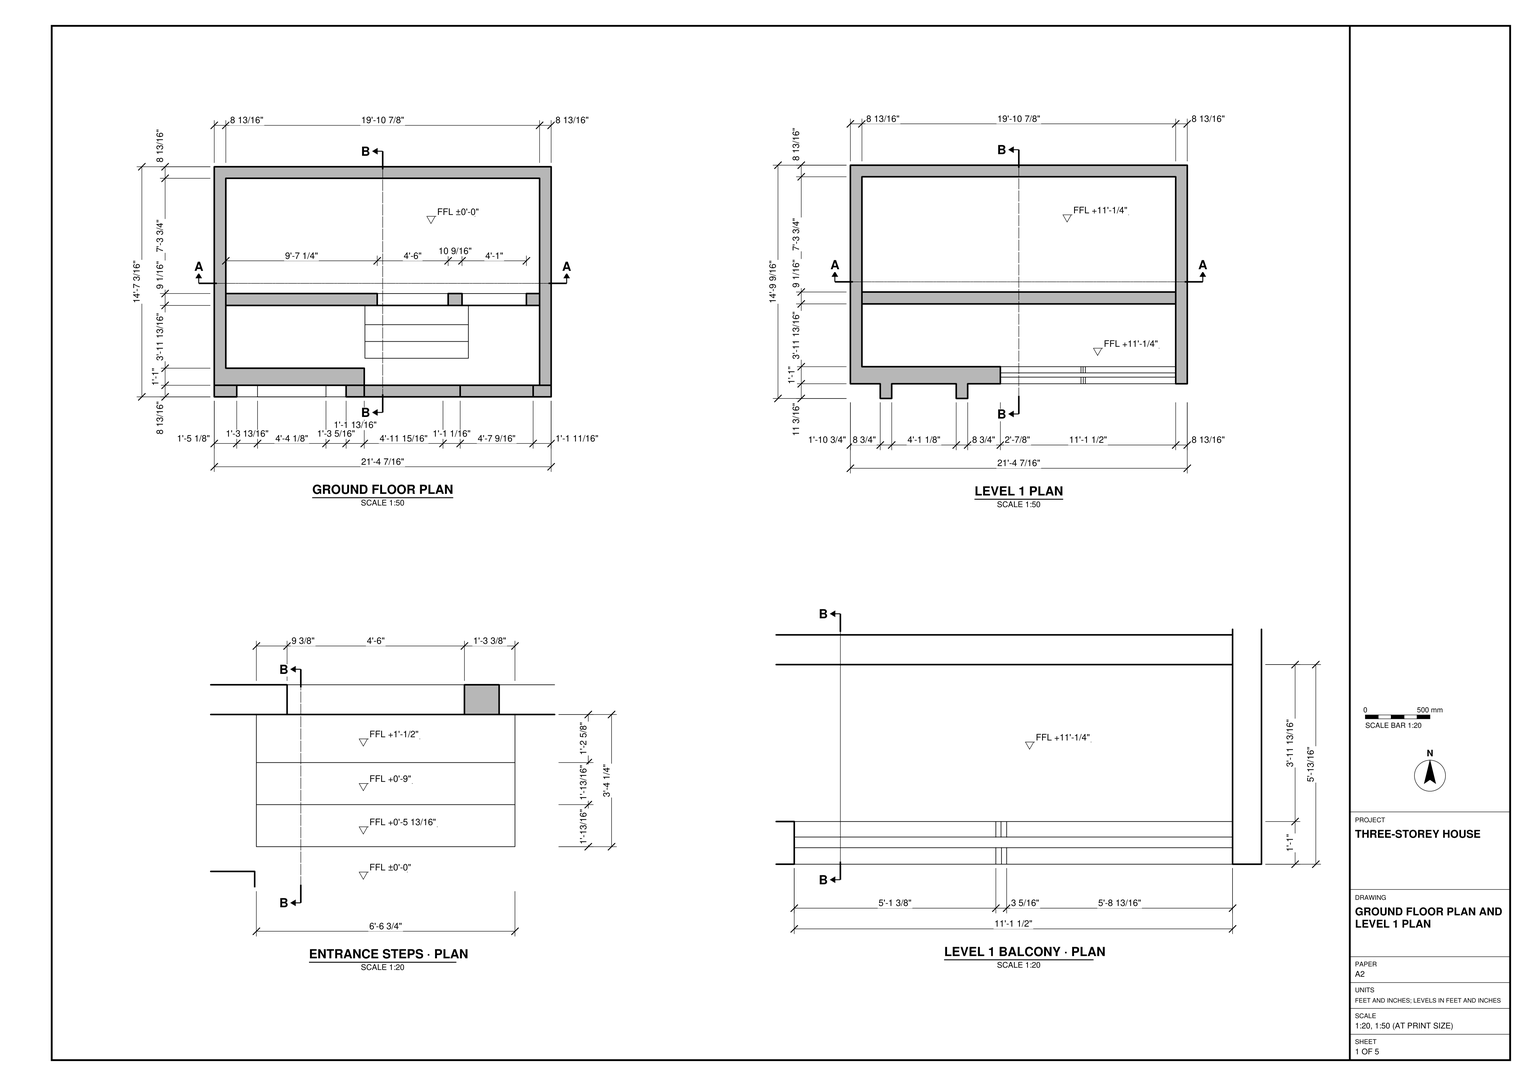
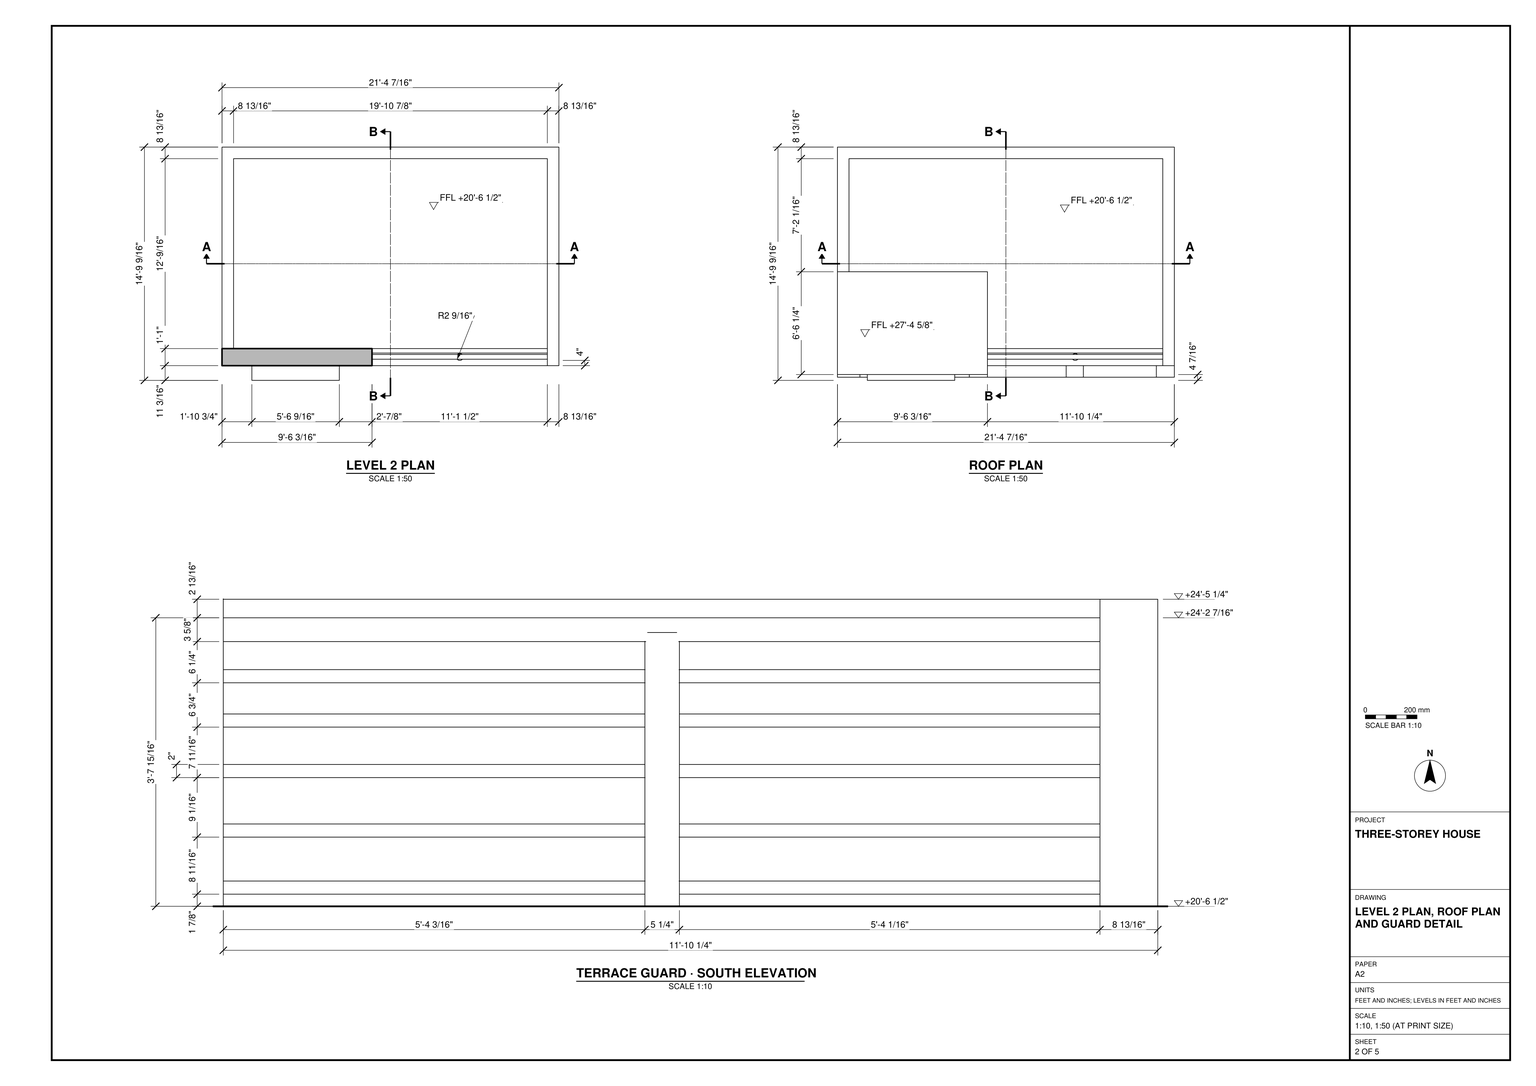
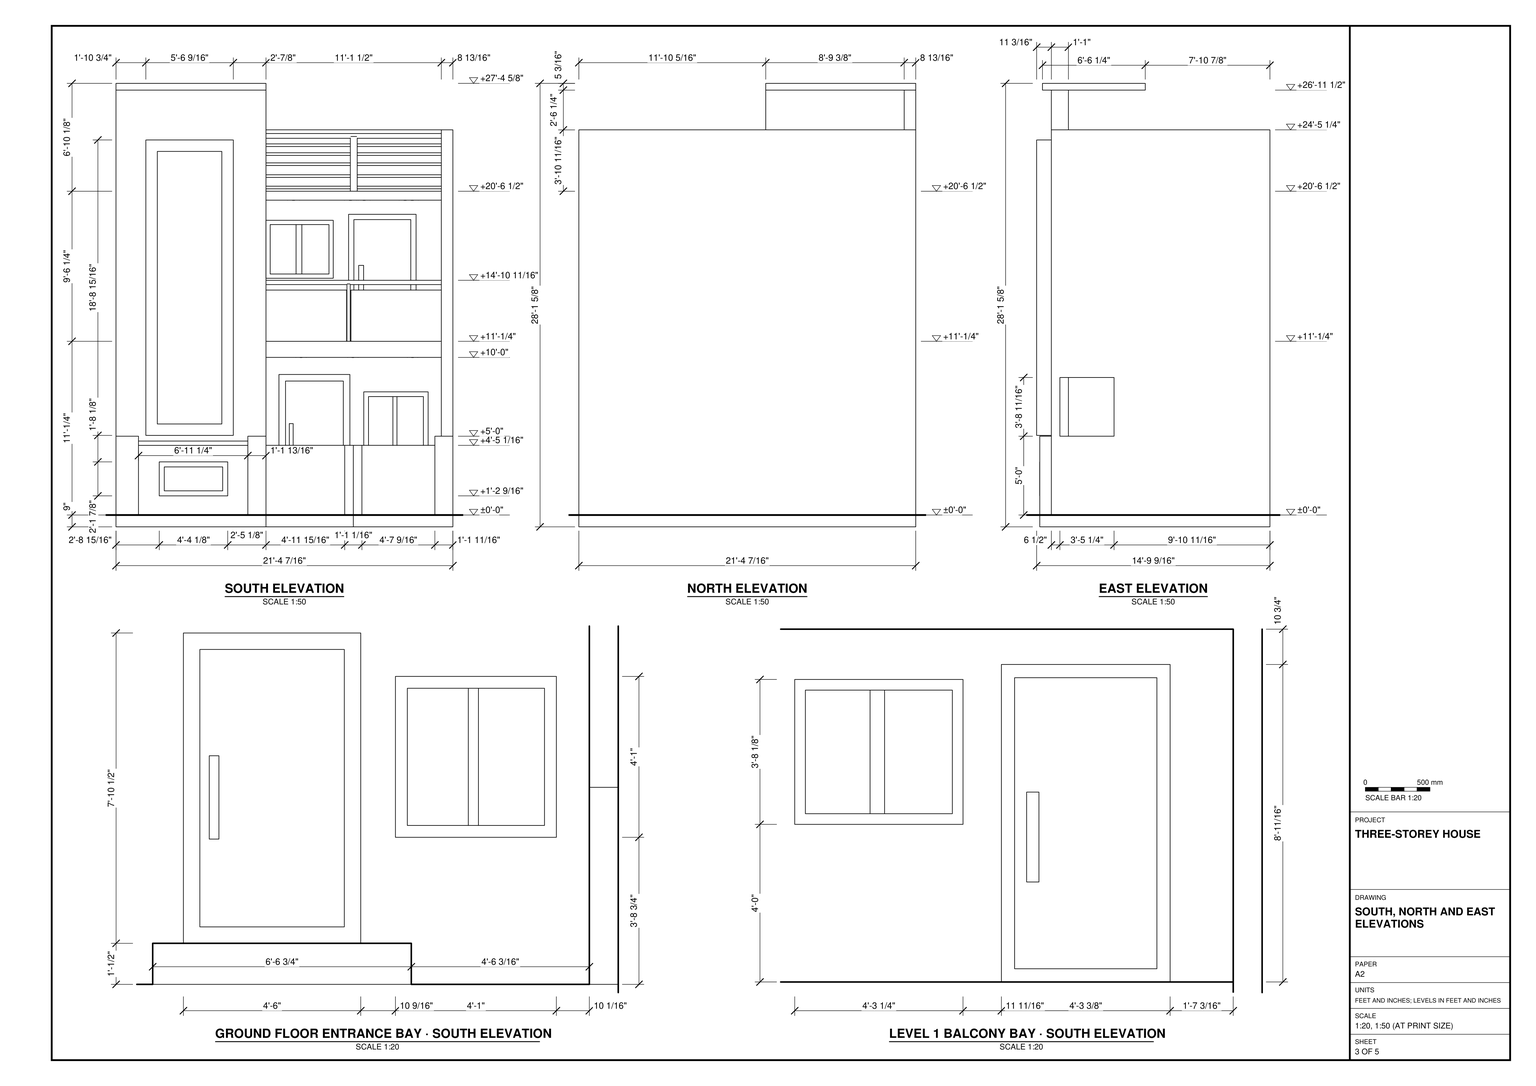
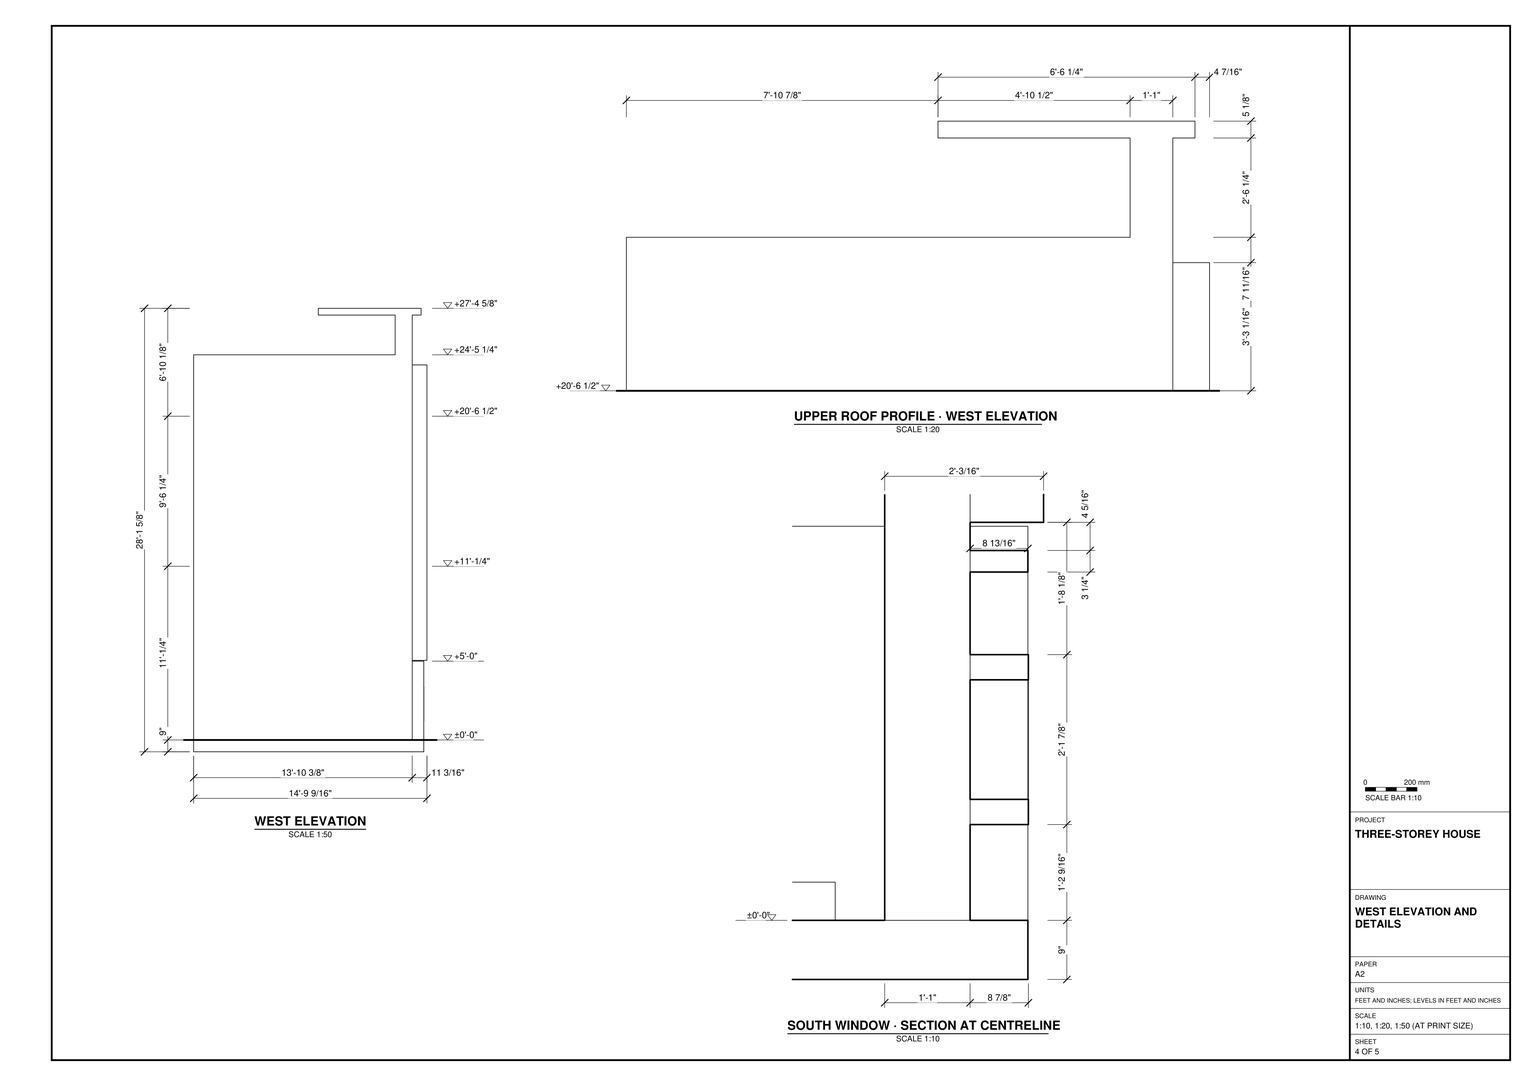
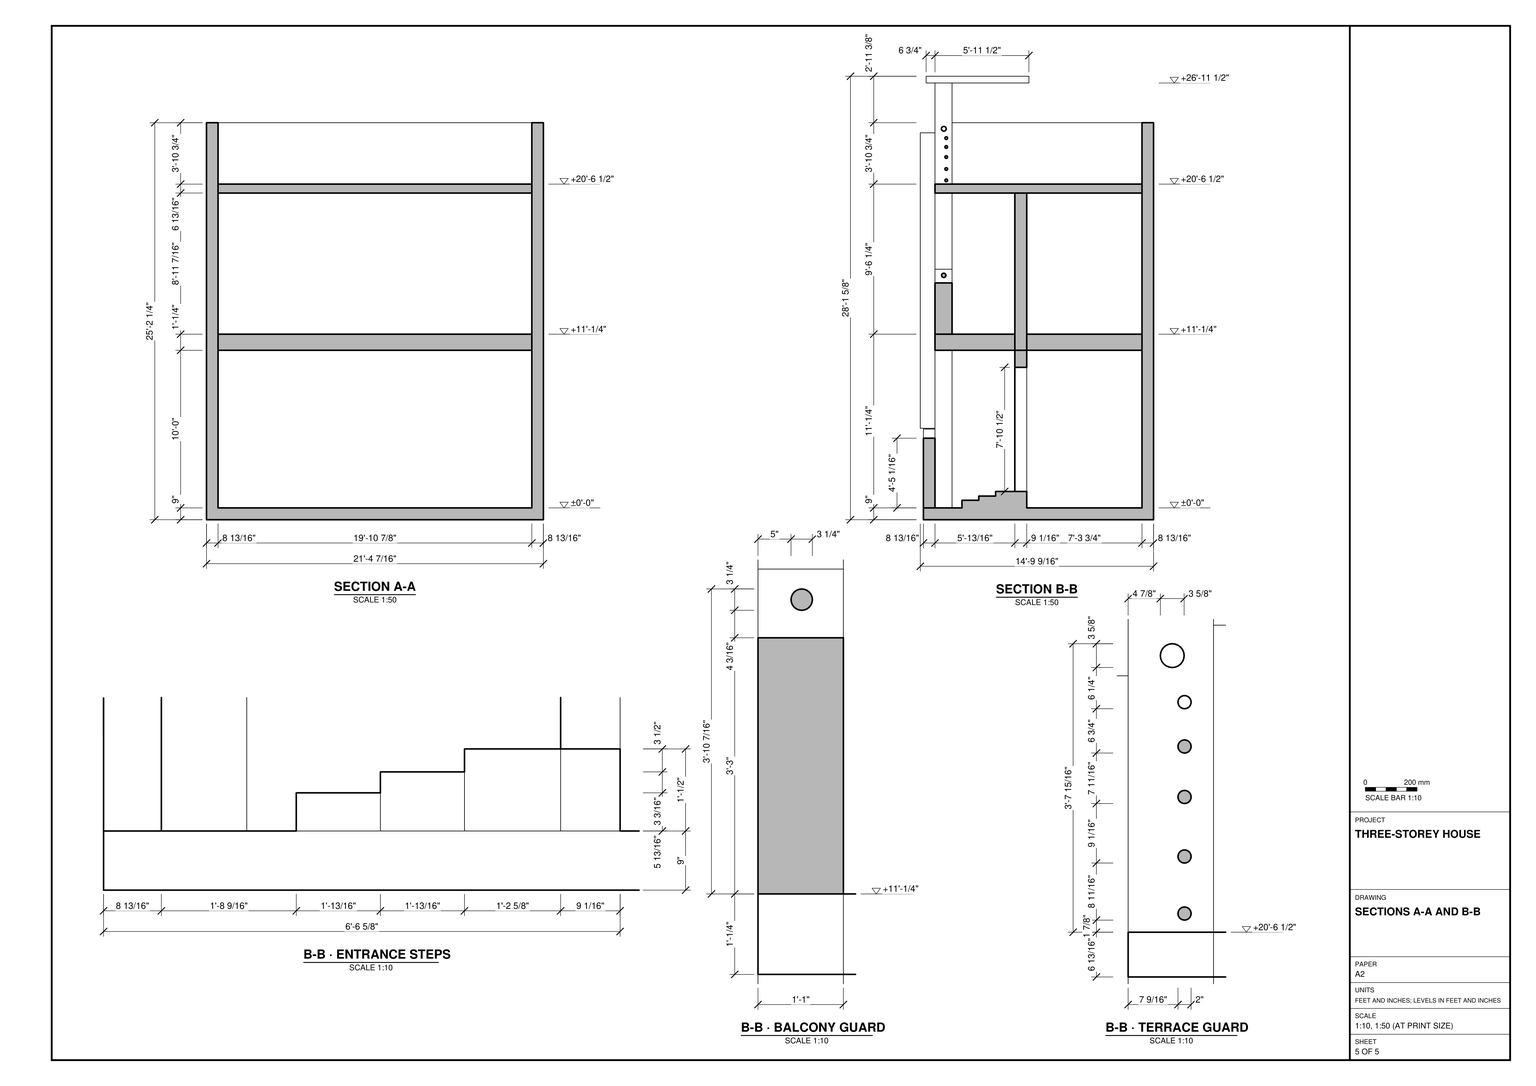
Build the residence in SketchUp from task_files/diagram_01.pdf. Work in feet and inches. Set the overall width along X to 21'-4 7/16", the depth along Y to 14'-9 9/16", and the height along Z to 28'-1 5/8". Use finished floor levels of ±0'-0", +11'-1/4", and +20'-6 1/2". Include the base below the ground-floor datum when setting the overall height.

Lay out the walls and slabs from the floor plans, using the wall thicknesses shown, including the 8 13/16" side walls. On the south face, distinguish the low front wall from the recessed entrance behind it. Model the broad entrance steps, the framed door and the adjacent divided window. Above the entrance, form the Level 1 balcony with its front guard, door and window. Match the tall framed panel on the left side of the south elevation. At Level 2, model the terrace, its perimeter walls, the horizontal rails across the south opening and the raised flat roof over the front-left portion of the terrace.

Include built-in joinery and main furniture where shown. Keep walls, slabs, roof elements and individual furniture or joinery pieces in separate groups or components, and use components for repeated parts. Decor and loose items may be any suitable library components. Save one SketchUp model as output_files/three_storey_residence_with_a_balcony_and_roof_terrace.skp.

# SketchUp Ruby script. Lengths in inches.
U = 1.inch
M = Sketchup.active_model
def pt(a) = Geom::Point3d.new(a.map { |v| v * U })
def face(e, loops, mat)
  f = e.add_face(loops[0].map { |a| pt(a) })
  loops[1..].each { |l| e.add_face(l.map { |a| pt(a) }).erase! }
  f.material = f.back_material = mat if mat
  f
end
# faces: each face lists its corners as indices into pts; further lists are holes
def faces(e, pts, list, mat = nil) = list.each { |f| face(e, (f[0].is_a?(Array) ? f : [f]).map { |l| l.map { |i| pts[i] } }, mat) }
# xy, xz, yz: faces in a plane at the given z, y or x. An outline is a flat list of corners, or four numbers for a rectangle; further outlines are holes
def ring(l) = l.size == 4 ? [[l[0], l[1]], [l[2], l[1]], [l[2], l[3]], [l[0], l[3]]] : l.each_slice(2).to_a
def flat(e, list, mat, &to3) = list.each { |f| face(e, (f[0].is_a?(Array) ? f : [f]).map { |l| ring(l).map { |u, v| to3.(u, v) } }, mat) }
def xy(e, z, list, mat = nil) = flat(e, list, mat) { |x, y| [x, y, z] }
def xz(e, y, list, mat = nil) = flat(e, list, mat) { |x, z| [x, y, z] }
def yz(e, x, list, mat = nil) = flat(e, list, mat) { |y, z| [x, y, z] }
def lines(e, pts, list) = list.each { |a, b| e.add_line(pt(pts[a]), pt(pts[b])) }
# prism: a flat outline (further loops are holes) pulled along v
def prism(e, loops, v, mat = nil)
  f = face(e, loops, mat); d = Geom::Vector3d.new(v.map { |x| x * U })
  f.pushpull(f.normal.samedirection?(d) ? d.length : -d.length)
end
def box(e, o, s, mat = nil) = prism(e, [[o, [o[0] + s[0], o[1], o[2]], [o[0] + s[0], o[1] + s[1], o[2]], [o[0], o[1] + s[1], o[2]]]], [0, 0, s[2]], mat)
def at(x, y, z, deg = 0) = Geom::Transformation.translation(pt([x, y, z])) * Geom::Transformation.rotation(ORIGIN, Z_AXIS, deg.degrees)
def axes(o, x, y, z) = Geom::Transformation.new([*x, 0, *y, 0, *z, 0, *pt(o).to_a, 1])
def part(name) = M.definitions.add(name)
# library, detail: a bought-in or finely detailed component or shape, given as its bounding box
def library(name, o, s) = part(name).tap { |d| box(d.entities, o, s) }
def detail(e, o, s) = box(e.add_group.entities, o, s)
def put(e, d, t, mat = nil) = e.add_instance(d, t).tap { |i| i.material = mat if mat }
def group(e, t, mat = nil) = e.add_group.tap { |g| g.transformation = t; g.material = mat if mat }.entities
root = M.entities
M.materials.add("[Asphalt New]").color = [67, 60, 62]
M.materials.add("[Color C03]").color = [255, 178, 101]
M.materials.add("[Color M07]").color = [58, 58, 58]
M.materials.add("[Color M08]").color = [30, 30, 30]
M.materials.add("[Formica Beige]").color = [211, 187, 149]
M.materials.add("[Formica Graystone]").color = [149, 146, 135]
M.materials.add("[Formica Speckled Grey]").color = [94, 105, 111]
M.materials.add("[Marble Carrara Gold Floor Tile]").color = [225, 223, 217]
M.materials.add("[Terrazzo Light Blue]").color = [196, 214, 227]
M.materials.add("[Translucent Glass Safety]").color = [204, 235, 244]
M.materials["[Translucent Glass Safety]"].alpha = 0.5
M.materials.add("[Window Covering 01]").color = [169, 163, 146]
M.materials.add("[Wood Bamboo]").color = [177, 105, 43]
M.materials.add("[Wood Floor Parquet]").color = [145, 89, 39]
M.materials.add("[Wood Veneer 01]").color = [63, 37, 19]
c1 = library("Group\#1",[-0.5,-0.5,-0.1],[9.125,9.125,0.2])
c2 = library("Group\#2",[-0.5,-0.5,-0.1],[9.125,9.125,0.2])
c3 = library("Group\#3",[-0.5,-0.5,-0.1],[9.125,9.125,0.2])
c4 = library("Group\#4",[-0.5,-0.5,-0.1],[9.125,9.125,0.2])
c5 = library("Group\#5",[-0.5,-0.5,-0.1],[9.125,9.125,0.2])
c6 = library("Group\#6",[-0.5,-0.5,-0.1],[9.125,9.125,0.2])
c7 = library("Group\#7",[-0.5,-0.5,-0.1],[7.875,7.875,0.2])
c8 = library("Group\#8",[-0.5,-0.5,-0.1],[7.875,7.875,0.2])
c9 = library("Group\#9",[-0.5,-0.5,-0.1],[7.875,7.875,0.2])
c10 = library("Group\#10",[-0.5,-0.5,-0.1],[7.875,7.875,0.2])
c11 = library("Group\#11",[-0.5,-0.5,-0.1],[7.875,7.875,0.2])
c12 = library("Group\#12",[-0.5,-0.5,-0.1],[7.875,7.875,0.2])
xy(root,0,[[0,2.39,256.47,177.57]])
xy(root,9,[[0,2.39,17.125,11.1875],[100.375,2.39,114.1875,11.1875],[114.1875,2.39,174.13,11.1875],[187.21,2.39,242.76,11.1875],[242.76,2.39,256.47,11.1875],
  [114.1875,11.1875,247.66,11.1875,247.66,71.98,193.45,71.98,193.45,31.73,114.7,31.73,114.7,71.98,8.8,71.98,8.8,24.1875,114.1875,24.1875],[8.8,81.03,247.66,168.77]])
xy(root,9,[[17.125,2.39,100.375,11.1875]],"[Color C03]")
xy(root,14.8125,[[114.7,31.73,193.45,44.53]],"[Terrazzo Light Blue]")
xy(root,18,[[114.7,44.53,193.45,57.34]],"[Terrazzo Light Blue]")
xy(root,21.5,[[124.06,71.98,178.06,81.03]])
xy(root,21.5,[[114.7,57.34,193.45,71.98]],"[Terrazzo Light Blue]")
xy(root,23.58,[[32.93,2.3125,85.06,11.1875]],"[Formica Speckled Grey]")
xy(root,27.42,[[36.77,2.3125,81.22,11.1875]],"[Formica Speckled Grey]")
xy(root,45.62,[[36.77,2.3125,81.22,11.1875]],"[Formica Speckled Grey]")
xy(root,49.46,[[32.93,2.3125,85.06,11.1875]],"[Formica Speckled Grey]")
xy(root,53.78,[[188.62,71.98,237.62,81.03]])
xy(root,62.03,[[17.125,2.39,100.375,11.1875]])
xy(root,62.06,[[174.13,2.39,187.21,11.1875]],"[Color M08]")
xy(root,62.06,[[114.1875,2.39,174.13,11.1875],[187.21,2.39,242.76,11.1875]],"[Wood Floor Parquet]")
xy(root,65.3125,[[17.125,2.39,100.375,11.1875]],"[Color C03]")
xy(root,69,[[0,2.39,17.125,11.1875],[100.375,2.39,114.1875,11.1875],[242.76,2.39,256.47,11.1875]],"[Color C03]")
xy(root,69,[[247.66,17.7,256.47,58.91]],"[Formica Speckled Grey]")
xy(root,69.6,[[22.74,0,89.3,11.1875]],"[Asphalt New]")
xy(root,78.33,[[31.47,0,80.58,11.1875]],"[Wood Bamboo]")
xy(root,102.78,[[188.62,71.98,237.62,81.03]])
xy(root,113.7,[[247.66,17.7,256.47,58.91]],"[Formica Speckled Grey]")
xy(root,116,[[124.06,71.98,178.06,81.03]])
xy(root,129,[[114.1875,11.1875,114.1875,24.1875,8.8,24.1875,8.8,71.98,247.66,71.98,247.66,11.1875],[8.8,71.98,247.66,81.03],[8.8,81.03,247.66,168.77]])
xy(root,141.25,[[114.1875,11.1875,175.58,24.1875],[175.58,11.1875,177.3,11.1875,177.3,16.46,176.97,16.4375,176.65,16.5,176.36,16.65,176.12,16.87,175.9375,17.14,175.83,17.45,175.82,17.77,175.88,18.09,176.03,18.39,176.25,18.63,176.52,18.81,176.83,18.91,177.15,18.93,177.15,24.1875,175.58,24.1875],[177.3,11.1875,178.875,11.1875,178.875,24.1875,177.15,24.1875,177.15,18.93,177.47,18.86,177.76,18.72,178.01,18.5,178.1875,18.23,178.29,17.92,178.31,17.59,178.24,17.27,178.1,16.98,177.88,16.74,177.61,16.56,177.3,16.46],[178.875,11.1875,247.66,24.1875],[176.97,16.4375,176.65,16.5,176.36,16.65,176.12,16.87,175.9375,17.14,175.83,17.45,175.82,17.77,175.88,18.09,176.03,18.39,176.25,18.63,176.52,18.81,176.83,18.91,177.15,18.93,177.47,18.86,177.76,18.72,178.01,18.5,178.1875,18.23,178.29,17.92,178.31,17.59,178.24,17.27,178.1,16.98,177.88,16.74,177.61,16.56,177.3,16.46],
  [8.8,24.1875,247.66,71.98],[8.8,81.03,247.66,168.77]])
xy(root,180.25,[[114.1875,11.1875,175.58,24.1875],[178.875,11.1875,247.66,24.1875]])
xy(root,184.9375,[[176.97,16.4375,177.3,16.46,177.61,16.56,177.88,16.74,178.1,16.98,178.24,17.27,178.31,17.59,178.29,17.92,178.1875,18.23,178.01,18.5,177.76,18.72,177.47,18.86,177.15,18.93,176.83,18.91,176.52,18.81,176.25,18.63,176.03,18.39,175.88,18.09,175.82,17.77,175.83,17.45,175.9375,17.14,176.12,16.87,176.36,16.65,176.65,16.5]])
xy(root,248.6875,[[114.1875,11.1875,114.1875,24.1875,8.8,24.1875,8.8,71.98,247.66,71.98,247.66,11.1875],[8.8,71.98,247.66,81.03],[8.8,81.03,247.66,168.77]])
xy(root,255.5,[[[114.1875,11.1875,247.66,24.1875],[181.01,15.17,180.33,15.26,179.69,15.52,179.15,15.94,178.73,16.48,178.47,17.12,178.38,17.8,178.47,18.48,178.73,19.11,179.15,19.65,179.69,20.07,180.33,20.33,181.01,20.42,181.6875,20.33,182.32,20.07,182.86,19.65,183.28,19.11,183.54,18.48,183.63,17.8,183.54,17.12,183.28,16.48,182.86,15.94,182.32,15.52,181.6875,15.26]]],"[Color C03]")
xy(root,255.5,[[8.8,24.1875,247.66,168.77]],"[Formica Graystone]")
xy(root,285.8125,[[31.47,0,80.58,11.1875]],"[Wood Bamboo]")
xy(root,294.54,[[22.74,0,89.3,11.1875]],"[Asphalt New]")
xy(root,297.1875,[[181.01,15.17,181.6875,15.26,182.32,15.52,182.86,15.94,183.28,16.48,183.54,17.12,183.63,17.8,183.54,18.48,183.28,19.11,182.86,19.65,182.32,20.07,181.6875,20.33,181.01,20.42,180.33,20.33,179.69,20.07,179.15,19.65,178.73,19.11,178.47,18.48,178.38,17.8,178.47,17.12,178.73,16.48,179.15,15.94,179.69,15.52,180.33,15.26]])
xy(root,302.25,[[247.66,11.1875,256.47,11.1875,256.47,177.57,0,177.57,0,24.1875,8.8,24.1875,8.8,168.77,247.66,168.77]],"[Formica Speckled Grey]")
xy(root,332.49,[[0,4.4375,114.1875,11.1875],[0,24.1875,8.8,82.6875],[8.8,24.1875,114.1875,82.6875]])
xy(root,337.625,[[0,4.4375,114.1875,82.6875]],"[Formica Beige]")
xz(root,0,[[[22.74,69.6,89.3,294.54],[31.47,78.33,80.58,285.8125]]],"[Asphalt New]")
xz(root,2.3125,[[[32.93,23.58,85.06,49.46],[36.77,27.42,81.22,45.62]]],"[Formica Speckled Grey]")
xz(root,2.39,[[0,0,114.1875,9],[0,9,17.125,69],[100.375,9,114.1875,69],[242.76,9,256.47,69],[17.125,62.03,100.375,65.3125]],"[Color C03]")
xz(root,2.39,[[114.1875,0,180.67,0,180.67,62.06,174.13,62.06,174.13,9,114.1875,9],[180.67,0,256.47,0,256.47,9,187.21,9,187.21,62.06,180.67,62.06]],"[Color M08]")
xz(root,2.39,[[114.1875,9,174.13,62.06],[187.21,9,242.76,62.06]],"[Wood Floor Parquet]")
xz(root,4.4375,[[0,332.49,114.1875,337.625]],"[Formica Speckled Grey]")
xz(root,11.1875,[[0,9,8.8,69],[8.8,9,17.125,69],[100.375,9,114.1875,69],[242.76,9,247.66,69],[247.66,9,256.47,69]])
xz(root,11.1875,[[[17.125,9,100.375,62.03],[32.93,23.58,85.06,49.46]],[[17.125,65.3125,100.375,65.3125,100.375,69,114.1875,69,114.1875,332.49,0,332.49,0,69,17.125,69],[22.74,69.6,89.3,294.54]],[114.1875,129,247.66,141.25],[114.1875,248.6875,247.66,255.5]],"[Color C03]")
xz(root,11.1875,[[174.13,9,187.21,62.06]],"[Color M08]")
xz(root,11.1875,[[36.77,27.42,81.22,45.62],[247.66,69,256.47,302.25]],"[Formica Speckled Grey]")
xz(root,11.1875,[[114.1875,141.25,175.58,180.25],[178.875,141.25,247.66,180.25]],"[Translucent Glass Safety]")
xz(root,11.1875,[[31.47,78.33,80.58,285.8125]],"[Wood Bamboo]")
xz(root,11.1875,[[114.1875,9,174.13,62.06],[187.21,9,242.76,62.06]],"[Wood Floor Parquet]")
xz(root,17.7,[[247.66,69,256.47,113.7]],"[Formica Speckled Grey]")
xz(root,24.1875,[[8.8,129,114.1875,141.25],[8.8,141.25,114.1875,248.6875],[8.8,248.6875,114.1875,255.5]])
xz(root,24.1875,[[8.8,255.5,114.1875,332.49]],"[Formica Graystone]")
xz(root,24.1875,[[8.8,9,114.1875,129],[0,302.25,8.8,332.49]],"[Formica Speckled Grey]")
xz(root,24.1875,[[114.1875,141.25,175.58,180.25],[178.875,141.25,247.66,180.25]],"[Translucent Glass Safety]")
xz(root,31.73,[[114.7,9,193.45,14.8125]])
xz(root,44.53,[[114.7,14.8125,193.45,18]],"[Terrazzo Light Blue]")
xz(root,57.34,[[114.7,18,193.45,21.5]],"[Terrazzo Light Blue]")
xz(root,58.91,[[247.66,69,256.47,113.7]],"[Formica Speckled Grey]")
xz(root,71.98,[[8.8,129,247.66,141.25]])
xz(root,71.98,[[131.93,53.24,134.87,78.61],[184.76,171.7,188.51,199.07]],"[Formica Speckled Grey]")
xz(root,71.98,[[[8.8,9,114.7,9,114.7,21.5,124.06,21.5,124.06,116,178.06,116,178.06,21.5,193.45,21.5,193.45,9,247.66,9,247.66,129,8.8,129],[188.62,53.78,237.62,102.78]],[[8.8,141.25,177.07,141.25,177.07,237.9375,228.45,237.9375,228.45,141.25,247.66,141.25,247.66,248.6875,8.8,248.6875],[114.14,189.25,165.39,233.375]]],"[Marble Carrara Gold Floor Tile]")
xz(root,71.98,[[192.24,57.39,210.81,99.16],[213.89,57.39,234.01,99.16],[117.38,192.5,137.08,230.125],[141.5,192.5,162.14,230.125]],"[Window Covering 01]")
xz(root,71.98,[[[124.06,21.5,178.06,116],[129.0625,26.5,173.05,110.99]],[[129.0625,26.5,173.05,110.99],[131.93,53.24,134.87,78.61]],[[181.1,145.27,224.42,233.91],[184.76,171.7,188.51,199.07]]],"[Wood Bamboo]")
xz(root,71.98,[[[188.62,53.78,237.62,102.78],[192.24,57.39,234.01,99.16]],[210.81,57.39,213.89,99.16],[[177.07,141.25,228.45,237.9375],[181.1,145.27,224.42,233.91]],[[114.14,189.25,165.39,233.375],[117.38,192.5,162.14,230.125]],[137.08,192.5,141.5,230.125]],"[Wood Veneer 01]")
xz(root,81.03,[[[8.8,9,247.66,129],[124.06,21.5,178.06,116],[188.62,53.78,237.62,102.78]],[8.8,129,247.66,141.25],[8.8,141.25,247.66,248.6875]])
xz(root,82.6875,[[0,332.49,114.1875,337.625]],"[Formica Speckled Grey]")
xz(root,168.77,[[8.8,9,247.66,129],[8.8,129,247.66,141.25],[8.8,141.25,247.66,248.6875],[8.8,248.6875,247.66,255.5]])
xz(root,168.77,[[8.8,255.5,247.66,302.25]],"[Formica Graystone]")
xz(root,177.57,[[0,0,256.47,9],[0,9,256.47,302.25]],"[Formica Speckled Grey]")
yz(root,0,[[2.39,0,177.57,9],[2.39,9,11.1875,69],[11.1875,9,11.1875,332.49,4.4375,332.49,4.4375,337.625,82.6875,337.625,82.6875,332.49,24.1875,332.49,24.1875,302.25,177.57,302.25,177.57,9]],"[Formica Speckled Grey]")
yz(root,8.8,[[71.98,9,81.03,129],[81.03,9,168.77,129],[24.1875,129,71.98,141.25],[71.98,129,81.03,248.6875],[81.03,129,168.77,141.25],
  [81.03,141.25,168.77,248.6875],[24.1875,248.6875,71.98,255.5],[71.98,248.6875,81.03,255.5],[81.03,248.6875,168.77,255.5]])
yz(root,8.8,[[24.1875,255.5,168.77,302.25]],"[Formica Graystone]")
yz(root,8.8,[[24.1875,9,71.98,129],[24.1875,141.25,71.98,248.6875]],"[Marble Carrara Gold Floor Tile]")
yz(root,17.125,[[2.39,62.03,11.1875,65.3125]])
yz(root,17.125,[[2.39,9,11.1875,62.03],[2.39,65.3125,11.1875,69]],"[Color C03]")
yz(root,22.74,[[0,69.6,11.1875,294.54]],"[Asphalt New]")
yz(root,31.47,[[0,78.33,11.1875,285.8125]],"[Wood Bamboo]")
yz(root,32.93,[[2.3125,23.58,11.1875,49.46]],"[Formica Speckled Grey]")
yz(root,36.77,[[2.3125,27.42,11.1875,45.62]],"[Formica Speckled Grey]")
yz(root,80.58,[[0,78.33,11.1875,285.8125]],"[Wood Bamboo]")
yz(root,81.22,[[2.3125,27.42,11.1875,45.62]],"[Formica Speckled Grey]")
yz(root,85.06,[[2.3125,23.58,11.1875,49.46]],"[Formica Speckled Grey]")
yz(root,89.3,[[0,69.6,11.1875,294.54]],"[Asphalt New]")
yz(root,100.375,[[2.39,62.03,11.1875,65.3125]])
yz(root,100.375,[[2.39,9,11.1875,62.03],[2.39,65.3125,11.1875,69]],"[Color C03]")
yz(root,114.1875,[[2.39,9,11.1875,62.06],[11.1875,129,24.1875,141.25],[11.1875,141.25,24.1875,180.25],[[11.1875,180.25,24.1875,190.71],[17.84,184.44,17.42,184.49,17.03,184.65,16.69,184.91,16.43,185.25,16.27,185.64,16.22,186.06,16.27,186.48,16.43,186.87,16.69,187.21,17.03,187.47,17.42,187.63,17.84,187.69,18.26,187.63,18.65,187.47,18.99,187.21,19.25,186.87,19.41,186.48,19.47,186.06,19.41,185.64,19.25,185.25,18.99,184.91,18.65,184.65,18.26,184.49]],[17.84,184.44,17.42,184.49,17.03,184.65,16.69,184.91,16.43,185.25,16.27,185.64,16.22,186.06,16.27,186.48,16.43,186.87,16.69,187.21,17.03,187.47,17.42,187.63,17.84,187.69,18.26,187.63,18.65,187.47,18.99,187.21,19.25,186.87,19.41,186.48,19.47,186.06,19.41,185.64,19.25,185.25,18.99,184.91,18.65,184.65,18.26,184.49],
  [11.1875,248.6875,24.1875,255.5]])
yz(root,114.1875,[[11.1875,9,24.1875,129],[2.39,62.06,11.1875,69],[11.1875,190.71,24.1875,248.6875],[[11.1875,255.5,24.1875,332.49],[17.9,295.8,17.43,295.86,17,296.05,16.62,296.33,16.33,296.71,16.15,297.15,16.09,297.62,16.15,298.08,16.33,298.52,16.62,298.9,17,299.19,17.43,299.37,17.9,299.43,18.37,299.37,18.81,299.19,19.18,298.9,19.47,298.52,19.65,298.08,19.71,297.62,19.65,297.15,19.47,296.71,19.18,296.33,18.81,296.05,18.37,295.86],[19.77,289.53,19.52,289.57,19.27,289.67,19.07,289.83,18.91,290.03,18.81,290.27,18.77,290.53,18.81,290.79,18.91,291.03,19.07,291.24,19.27,291.4,19.52,291.5,19.77,291.53,20.03,291.5,20.27,291.4,20.48,291.24,20.64,291.03,20.74,290.79,20.77,290.53,20.74,290.27,20.64,290.03,20.48,289.83,20.27,289.67,20.03,289.57],[19.77,282.78,19.52,282.82,19.27,282.92,19.07,283.08,18.91,283.28,18.81,283.52,18.77,283.78,18.81,284.04,18.91,284.28,19.07,284.49,19.27,284.65,19.52,284.75,19.77,284.78,20.03,284.75,20.27,284.65,20.48,284.49,20.64,284.28,20.74,284.04,20.77,283.78,20.74,283.52,20.64,283.28,20.48,283.08,20.27,282.92,20.03,282.82],[19.77,275.09,19.52,275.13,19.27,275.23,19.07,275.39,18.91,275.59,18.81,275.84,18.77,276.09,18.81,276.35,18.91,276.59,19.07,276.8,19.27,276.96,19.52,277.0625,19.77,277.09,20.03,277.0625,20.27,276.96,20.48,276.8,20.64,276.59,20.74,276.35,20.77,276.09,20.74,275.84,20.64,275.59,20.48,275.39,20.27,275.23,20.03,275.13],[19.77,266.03,19.52,266.07,19.27,266.17,19.07,266.33,18.91,266.53,18.81,266.77,18.77,267.03,18.81,267.29,18.91,267.53,19.07,267.74,19.27,267.9,19.52,268,19.77,268.03,20.03,268,20.27,267.9,20.48,267.74,20.64,267.53,20.74,267.29,20.77,267.03,20.74,266.77,20.64,266.53,20.48,266.33,20.27,266.17,20.03,266.07],[19.77,257.34,19.52,257.38,19.27,257.48,19.07,257.64,18.91,257.84,18.81,258.09,18.77,258.34,18.81,258.6,18.91,258.84,19.07,259.05,19.27,259.21,19.52,259.3125,19.77,259.34,20.03,259.3125,20.27,259.21,20.48,259.05,20.64,258.84,20.74,258.6,20.77,258.34,20.74,258.09,20.64,257.84,20.48,257.64,20.27,257.48,20.03,257.38]]],"[Color C03]")
yz(root,114.1875,[[4.4375,332.49,82.6875,337.625]],"[Formica Speckled Grey]")
yz(root,114.7,[[31.73,9,44.53,14.8125],[44.53,9,57.34,18],[57.34,9,71.98,21.5]],"[Terrazzo Light Blue]")
yz(root,124.06,[[71.98,21.5,81.03,116]])
yz(root,175.58,[[11.1875,141.25,24.1875,180.25]])
yz(root,178.06,[[71.98,21.5,81.03,116]])
yz(root,178.875,[[11.1875,141.25,24.1875,180.25]])
yz(root,187.21,[[2.39,9,11.1875,62.06]])
yz(root,188.62,[[71.98,53.78,81.03,102.78]])
yz(root,193.45,[[31.73,9,44.53,14.8125],[44.53,9,57.34,18],[57.34,9,71.98,21.5]],"[Terrazzo Light Blue]")
yz(root,237.62,[[71.98,53.78,81.03,102.78]])
yz(root,242.76,[[2.39,9,11.1875,62.06]])
yz(root,242.76,[[2.39,62.06,11.1875,69]],"[Color C03]")
yz(root,247.66,[[71.98,9,81.03,129],[81.03,9,168.77,129],[11.1875,129,71.98,141.25],[71.98,129,81.03,248.6875],[81.03,129,168.77,141.25],
  [11.1875,141.25,24.1875,180.25],[81.03,141.25,168.77,248.6875],[[11.1875,180.25,24.1875,190.71],[17.84,184.44,18.26,184.49,18.65,184.65,18.99,184.91,19.25,185.25,19.41,185.64,19.47,186.06,19.41,186.48,19.25,186.87,18.99,187.21,18.65,187.47,18.26,187.63,17.84,187.69,17.42,187.63,17.03,187.47,16.69,187.21,16.43,186.87,16.27,186.48,16.22,186.06,16.27,185.64,16.43,185.25,16.69,184.91,17.03,184.65,17.42,184.49]],[11.1875,248.6875,71.98,255.5],[71.98,248.6875,81.03,255.5],
  [81.03,248.6875,168.77,255.5]])
yz(root,247.66,[[24.1875,255.5,168.77,302.25]],"[Formica Graystone]")
yz(root,247.66,[[[11.1875,255.5,24.1875,302.25],[17.9,295.8,18.37,295.86,18.81,296.05,19.18,296.33,19.47,296.71,19.65,297.15,19.71,297.62,19.65,298.08,19.47,298.52,19.18,298.9,18.81,299.19,18.37,299.37,17.9,299.43,17.43,299.37,17,299.19,16.62,298.9,16.33,298.52,16.15,298.08,16.09,297.62,16.15,297.15,16.33,296.71,16.62,296.33,17,296.05,17.43,295.86],[19.77,289.53,20.03,289.57,20.27,289.67,20.48,289.83,20.64,290.03,20.74,290.27,20.77,290.53,20.74,290.79,20.64,291.03,20.48,291.24,20.27,291.4,20.03,291.5,19.77,291.53,19.52,291.5,19.27,291.4,19.07,291.24,18.91,291.03,18.81,290.79,18.77,290.53,18.81,290.27,18.91,290.03,19.07,289.83,19.27,289.67,19.52,289.57],[19.77,257.34,20.03,257.38,20.27,257.48,20.48,257.64,20.64,257.84,20.74,258.09,20.77,258.34,20.74,258.6,20.64,258.84,20.48,259.05,20.27,259.21,20.03,259.3125,19.77,259.34,19.52,259.3125,19.27,259.21,19.07,259.05,18.91,258.84,18.81,258.6,18.77,258.34,18.81,258.09,18.91,257.84,19.07,257.64,19.27,257.48,19.52,257.38],[19.77,282.78,20.03,282.82,20.27,282.92,20.48,283.08,20.64,283.28,20.74,283.52,20.77,283.78,20.74,284.04,20.64,284.28,20.48,284.49,20.27,284.65,20.03,284.75,19.77,284.78,19.52,284.75,19.27,284.65,19.07,284.49,18.91,284.28,18.81,284.04,18.77,283.78,18.81,283.52,18.91,283.28,19.07,283.08,19.27,282.92,19.52,282.82],[19.77,266.03,20.03,266.07,20.27,266.17,20.48,266.33,20.64,266.53,20.74,266.77,20.77,267.03,20.74,267.29,20.64,267.53,20.48,267.74,20.27,267.9,20.03,268,19.77,268.03,19.52,268,19.27,267.9,19.07,267.74,18.91,267.53,18.81,267.29,18.77,267.03,18.81,266.77,18.91,266.53,19.07,266.33,19.27,266.17,19.52,266.07],[19.77,275.09,20.03,275.13,20.27,275.23,20.48,275.39,20.64,275.59,20.74,275.84,20.77,276.09,20.74,276.35,20.64,276.59,20.48,276.8,20.27,276.96,20.03,277.0625,19.77,277.09,19.52,277.0625,19.27,276.96,19.07,276.8,18.91,276.59,18.81,276.35,18.77,276.09,18.81,275.84,18.91,275.59,19.07,275.39,19.27,275.23,19.52,275.13]]],"[Formica Speckled Grey]")
yz(root,247.66,[[11.1875,9,11.1875,129,71.98,129,71.98,69,58.91,69,58.91,113.7,17.7,113.7,17.7,69,71.98,69,71.98,9],[24.1875,141.25,24.1875,190.71,11.1875,190.71,11.1875,248.6875,71.98,248.6875,71.98,141.25]],"[Marble Carrara Gold Floor Tile]")
yz(root,256.47,[[[2.39,0,177.57,0,177.57,302.25,11.1875,302.25,11.1875,9,2.39,9],[17.7,69,58.91,113.7]],[2.39,9,11.1875,69]],"[Formica Speckled Grey]")
p = [[176.65,16.5,141.25],[176.97,16.4375,141.25],[176.97,16.4375,184.9375],[176.65,16.5,184.9375],[177.3,16.46,141.25],[177.3,16.46,184.9375],
  [176.36,16.65,141.25],[176.36,16.65,184.9375],[177.61,16.56,141.25],[177.61,16.56,184.9375],[176.12,16.87,141.25],[176.12,16.87,184.9375],
  [177.88,16.74,141.25],[177.88,16.74,184.9375],[178.1,16.98,141.25],[178.1,16.98,184.9375],[175.9375,17.14,141.25],[175.9375,17.14,184.9375],
  [178.24,17.27,141.25],[178.24,17.27,184.9375],[175.83,17.45,141.25],[175.83,17.45,184.9375],[178.31,17.59,141.25],[178.31,17.59,184.9375],
  [175.82,17.77,141.25],[175.82,17.77,184.9375],[178.29,17.92,141.25],[178.29,17.92,184.9375],[175.88,18.09,141.25],[175.88,18.09,184.9375],
  [178.1875,18.23,141.25],[178.1875,18.23,184.9375],[176.03,18.39,141.25],[176.03,18.39,184.9375],[178.01,18.5,141.25],[178.01,18.5,184.9375],
  [176.25,18.63,141.25],[176.25,18.63,184.9375],[177.76,18.72,141.25],[177.76,18.72,184.9375],[176.52,18.81,141.25],[176.52,18.81,184.9375],
  [177.47,18.86,141.25],[177.47,18.86,184.9375],[176.83,18.91,141.25],[176.83,18.91,184.9375],[177.15,18.93,141.25],[177.15,18.93,184.9375],
  [114.1875,17.42,184.49],[114.1875,17.84,184.44],[247.66,17.84,184.44],[247.66,17.42,184.49],[114.1875,18.26,184.49],[247.66,18.26,184.49],
  [114.1875,17.03,184.65],[247.66,17.03,184.65],[114.1875,18.65,184.65],[247.66,18.65,184.65],[114.1875,16.69,184.91],[247.66,16.69,184.91],
  [114.1875,18.99,184.91],[247.66,18.99,184.91],[114.1875,16.43,185.25],[247.66,16.43,185.25],[114.1875,19.25,185.25],[247.66,19.25,185.25],
  [114.1875,16.27,185.64],[247.66,16.27,185.64],[114.1875,19.41,185.64],[247.66,19.41,185.64],[114.1875,16.22,186.06],[247.66,16.22,186.06],
  [114.1875,19.47,186.06],[247.66,19.47,186.06],[114.1875,16.27,186.48],[247.66,16.27,186.48],[114.1875,19.41,186.48],[247.66,19.41,186.48],
  [114.1875,16.43,186.87],[247.66,16.43,186.87],[114.1875,19.25,186.87],[247.66,19.25,186.87],[114.1875,16.69,187.21],[247.66,16.69,187.21],
  [114.1875,18.99,187.21],[247.66,18.99,187.21],[114.1875,17.03,187.47],[247.66,17.03,187.47],[114.1875,18.65,187.47],[247.66,18.65,187.47],
  [114.1875,17.42,187.63],[247.66,17.42,187.63],[114.1875,18.26,187.63],[247.66,18.26,187.63],[114.1875,17.84,187.69],[247.66,17.84,187.69],
  [180.33,15.26,255.5],[181.01,15.17,255.5],[181.01,15.17,297.1875],[180.33,15.26,297.1875],[181.6875,15.26,255.5],[181.6875,15.26,297.1875],
  [179.69,15.52,255.5],[179.69,15.52,297.1875],[182.32,15.52,255.5],[182.32,15.52,297.1875],[179.15,15.94,255.5],[179.15,15.94,297.1875],
  [182.86,15.94,255.5],[182.86,15.94,297.1875],[178.73,16.48,255.5],[178.73,16.48,297.1875],[183.28,16.48,255.5],[183.28,16.48,297.1875],
  [178.47,17.12,255.5],[178.47,17.12,297.1875],[183.54,17.12,255.5],[183.54,17.12,297.1875],[178.38,17.8,255.5],[178.38,17.8,297.1875],
  [183.63,17.8,255.5],[183.63,17.8,297.1875],[178.47,18.48,255.5],[178.47,18.48,297.1875],[183.54,18.48,255.5],[183.54,18.48,297.1875],
  [178.73,19.11,255.5],[178.73,19.11,297.1875],[183.28,19.11,255.5],[183.28,19.11,297.1875],[179.15,19.65,255.5],[179.15,19.65,297.1875],
  [179.15,19.65,297.15],[182.86,19.65,255.5],[182.86,19.65,297.15],[182.86,19.65,297.1875],[179.69,20.07,255.5],[179.69,20.07,297.1875],
  [182.32,20.07,255.5],[182.32,20.07,297.1875],[180.33,20.33,255.5],[180.33,20.33,297.1875],[181.6875,20.33,255.5],[181.6875,20.33,297.1875],
  [181.01,20.42,255.5],[181.01,20.42,297.1875],[247.66,19.77,257.34],[247.66,19.52,257.38],[114.1875,19.52,257.38],[114.1875,19.77,257.34],
  [247.66,20.03,257.38],[114.1875,20.03,257.38],[247.66,19.27,257.48],[114.1875,19.27,257.48],[247.66,20.27,257.48],[114.1875,20.27,257.48],
  [247.66,19.07,257.64],[114.1875,19.07,257.64],[247.66,20.48,257.64],[114.1875,20.48,257.64],[247.66,18.91,257.84],[114.1875,18.91,257.84],
  [247.66,20.64,257.84],[114.1875,20.64,257.84],[247.66,18.81,258.09],[114.1875,18.81,258.09],[247.66,20.74,258.09],[114.1875,20.74,258.09],
  [247.66,18.77,258.34],[114.1875,18.77,258.34],[247.66,20.77,258.34],[114.1875,20.77,258.34],[247.66,18.81,258.6],[114.1875,18.81,258.6],
  [247.66,20.74,258.6],[114.1875,20.74,258.6],[247.66,18.91,258.84],[114.1875,18.91,258.84],[247.66,20.64,258.84],[114.1875,20.64,258.84],
  [247.66,19.07,259.05],[114.1875,19.07,259.05],[247.66,20.48,259.05],[114.1875,20.48,259.05],[247.66,19.27,259.21],[114.1875,19.27,259.21],
  [247.66,20.27,259.21],[114.1875,20.27,259.21],[247.66,19.52,259.3125],[114.1875,19.52,259.3125],[247.66,20.03,259.3125],[114.1875,20.03,259.3125],
  [247.66,19.77,259.34],[114.1875,19.77,259.34],[247.66,19.77,266.03],[247.66,19.52,266.07],[114.1875,19.52,266.07],[114.1875,19.77,266.03],
  [247.66,20.03,266.07],[114.1875,20.03,266.07],[247.66,19.27,266.17],[114.1875,19.27,266.17],[247.66,20.27,266.17],[114.1875,20.27,266.17],
  [247.66,19.07,266.33],[114.1875,19.07,266.33],[247.66,20.48,266.33],[114.1875,20.48,266.33],[247.66,18.91,266.53],[114.1875,18.91,266.53],
  [247.66,20.64,266.53],[114.1875,20.64,266.53],[247.66,18.81,266.77],[114.1875,18.81,266.77],[247.66,20.74,266.77],[114.1875,20.74,266.77],
  [247.66,18.77,267.03],[114.1875,18.77,267.03],[247.66,20.77,267.03],[114.1875,20.77,267.03],[247.66,18.81,267.29],[114.1875,18.81,267.29],
  [247.66,20.74,267.29],[114.1875,20.74,267.29],[247.66,18.91,267.53],[114.1875,18.91,267.53],[247.66,20.64,267.53],[114.1875,20.64,267.53],
  [247.66,19.07,267.74],[114.1875,19.07,267.74],[247.66,20.48,267.74],[114.1875,20.48,267.74],[247.66,19.27,267.9],[114.1875,19.27,267.9],
  [247.66,20.27,267.9],[114.1875,20.27,267.9],[247.66,19.52,268],[114.1875,19.52,268],[247.66,20.03,268],[114.1875,20.03,268],
  [247.66,19.77,268.03],[114.1875,19.77,268.03],[247.66,19.52,275.13],[247.66,19.27,275.23],[114.1875,19.27,275.23],[114.1875,19.52,275.13],
  [247.66,19.77,275.09],[114.1875,19.77,275.09],[247.66,20.03,275.13],[114.1875,20.03,275.13],[247.66,20.27,275.23],[114.1875,20.27,275.23],
  [247.66,19.07,275.39],[114.1875,19.07,275.39],[247.66,20.48,275.39],[114.1875,20.48,275.39],[247.66,18.91,275.59],[114.1875,18.91,275.59],
  [247.66,20.64,275.59],[114.1875,20.64,275.59],[247.66,18.81,275.84],[114.1875,18.81,275.84],[247.66,20.74,275.84],[114.1875,20.74,275.84],
  [247.66,18.77,276.09],[114.1875,18.77,276.09],[247.66,20.77,276.09],[114.1875,20.77,276.09],[247.66,18.81,276.35],[114.1875,18.81,276.35],
  [247.66,20.74,276.35],[114.1875,20.74,276.35],[247.66,18.91,276.59],[114.1875,18.91,276.59],[247.66,20.64,276.59],[114.1875,20.64,276.59],
  [247.66,19.07,276.8],[114.1875,19.07,276.8],[247.66,20.48,276.8],[114.1875,20.48,276.8],[247.66,19.27,276.96],[114.1875,19.27,276.96],
  [247.66,20.27,276.96],[114.1875,20.27,276.96],[247.66,19.52,277.0625],[114.1875,19.52,277.0625],[247.66,20.03,277.0625],[114.1875,20.03,277.0625],
  [247.66,19.77,277.09],[114.1875,19.77,277.09],[247.66,19.52,282.82],[247.66,19.27,282.92],[114.1875,19.27,282.92],[114.1875,19.52,282.82],
  [247.66,19.77,282.78],[114.1875,19.77,282.78],[247.66,20.03,282.82],[114.1875,20.03,282.82],[247.66,20.27,282.92],[114.1875,20.27,282.92],
  [247.66,19.07,283.08],[114.1875,19.07,283.08],[247.66,20.48,283.08],[114.1875,20.48,283.08],[247.66,18.91,283.28],[114.1875,18.91,283.28],
  [247.66,20.64,283.28],[114.1875,20.64,283.28],[247.66,18.81,283.52],[114.1875,18.81,283.52],[247.66,20.74,283.52],[114.1875,20.74,283.52],
  [247.66,18.77,283.78],[114.1875,18.77,283.78],[247.66,20.77,283.78],[114.1875,20.77,283.78],[247.66,18.81,284.04],[114.1875,18.81,284.04],
  [247.66,20.74,284.04],[114.1875,20.74,284.04],[247.66,18.91,284.28],[114.1875,18.91,284.28],[247.66,20.64,284.28],[114.1875,20.64,284.28],
  [247.66,19.07,284.49],[114.1875,19.07,284.49],[247.66,20.48,284.49],[114.1875,20.48,284.49],[247.66,19.27,284.65],[114.1875,19.27,284.65],
  [247.66,20.27,284.65],[114.1875,20.27,284.65],[247.66,19.52,284.75],[114.1875,19.52,284.75],[247.66,20.03,284.75],[114.1875,20.03,284.75],
  [247.66,19.77,284.78],[114.1875,19.77,284.78],[247.66,19.77,289.53],[247.66,19.52,289.57],[114.1875,19.52,289.57],[114.1875,19.77,289.53],
  [247.66,20.03,289.57],[114.1875,20.03,289.57],[247.66,19.27,289.67],[114.1875,19.27,289.67],[247.66,20.27,289.67],[114.1875,20.27,289.67],
  [247.66,19.07,289.83],[114.1875,19.07,289.83],[247.66,20.48,289.83],[114.1875,20.48,289.83],[247.66,18.91,290.03],[114.1875,18.91,290.03],
  [247.66,20.64,290.03],[114.1875,20.64,290.03],[247.66,18.81,290.27],[114.1875,18.81,290.27],[247.66,20.74,290.27],[114.1875,20.74,290.27],
  [247.66,18.77,290.53],[114.1875,18.77,290.53],[247.66,20.77,290.53],[114.1875,20.77,290.53],[247.66,18.81,290.79],[114.1875,18.81,290.79],
  [247.66,20.74,290.79],[114.1875,20.74,290.79],[247.66,18.91,291.03],[114.1875,18.91,291.03],[247.66,20.64,291.03],[114.1875,20.64,291.03],
  [247.66,19.07,291.24],[114.1875,19.07,291.24],[247.66,20.48,291.24],[114.1875,20.48,291.24],[247.66,19.27,291.4],[114.1875,19.27,291.4],
  [247.66,20.27,291.4],[114.1875,20.27,291.4],[247.66,19.52,291.5],[114.1875,19.52,291.5],[247.66,20.03,291.5],[114.1875,20.03,291.5],
  [247.66,19.77,291.53],[114.1875,19.77,291.53],[247.66,17.9,295.8],[247.66,17.43,295.86],[114.1875,17.43,295.86],[114.1875,17.9,295.8],
  [247.66,18.37,295.86],[114.1875,18.37,295.86],[247.66,17,296.05],[114.1875,17,296.05],[247.66,18.81,296.05],[114.1875,18.81,296.05],
  [247.66,16.62,296.33],[114.1875,16.62,296.33],[247.66,19.18,296.33],[114.1875,19.18,296.33],[247.66,16.33,296.71],[114.1875,16.33,296.71],
  [247.66,19.47,296.71],[114.1875,19.47,296.71],[247.66,16.15,297.15],[114.1875,16.15,297.15],[247.66,19.65,297.15],[114.1875,19.65,297.15],
  [247.66,16.09,297.62],[114.1875,16.09,297.62],[247.66,19.71,297.62],[114.1875,19.71,297.62],[247.66,16.15,298.08],[114.1875,16.15,298.08],
  [247.66,19.65,298.08],[114.1875,19.65,298.08],[247.66,16.33,298.52],[114.1875,16.33,298.52],[247.66,19.47,298.52],[114.1875,19.47,298.52],
  [247.66,16.62,298.9],[114.1875,16.62,298.9],[247.66,19.18,298.9],[114.1875,19.18,298.9],[247.66,17,299.19],[114.1875,17,299.19],
  [247.66,18.81,299.19],[114.1875,18.81,299.19],[247.66,17.43,299.37],[114.1875,17.43,299.37],[247.66,18.37,299.37],[114.1875,18.37,299.37],
  [247.66,17.9,299.43],[114.1875,17.9,299.43],[247.66,71.98,9],[256.47,71.98,9],[247.66,71.98,69],[256.47,71.98,69],
  [8.8,24.1875,9],[8.8,11.1875,9]]
faces(root,p,[[0,1,2,3],[1,4,5,2],[6,0,3,7],[4,8,9,5],[10,6,7,11],[8,12,13,9],[12,14,15,13],[16,10,11,17],
  [14,18,19,15],[20,16,17,21],[18,22,23,19],[24,20,21,25],[22,26,27,23],[28,24,25,29],[26,30,31,27],[32,28,29,33],
  [30,34,35,31],[36,32,33,37],[34,38,39,35],[40,36,37,41],[38,42,43,39],[44,40,41,45],[46,44,45,47],[42,46,47,43],
  [48,49,50,51],[49,52,53,50],[54,48,51,55],[52,56,57,53],[58,54,55,59],[56,60,61,57],[62,58,59,63],[60,64,65,61],
  [66,62,63,67],[64,68,69,65],[70,66,67,71],[68,72,73,69],[74,70,71,75],[72,76,77,73],[78,74,75,79],[76,80,81,77],
  [82,78,79,83],[80,84,85,81],[86,82,83,87],[84,88,89,85],[90,86,87,91],[88,92,93,89],[94,90,91,95],[92,94,95,93],
  [96,97,98,99],[97,100,101,98],[102,96,99,103],[100,104,105,101],[106,102,103,107],[104,108,109,105],[110,106,107,111],[108,112,113,109],
  [114,110,111,115],[112,116,117,113],[118,114,115,119],[116,120,121,117],[122,118,119,123],[120,124,125,121],[126,122,123,127],[124,128,129,125],
  [130,126,127,131,132],[128,133,134,135,129],[136,130,132,131,137],[133,138,139,135,134],[140,136,137,141],[138,142,143,139],[144,140,141,145],[142,144,145,143],
  [146,147,148,149],[150,146,149,151],[147,152,153,148],[154,150,151,155],[152,156,157,153],[158,154,155,159],[156,160,161,157],[162,158,159,163],
  [160,164,165,161],[166,162,163,167],[164,168,169,165],[170,166,167,171],[168,172,173,169],[174,170,171,175],[172,176,177,173],[178,174,175,179],
  [176,180,181,177],[182,178,179,183],[180,184,185,181],[186,182,183,187],[184,188,189,185],[190,186,187,191],[188,192,193,189],[192,190,191,193],
  [194,195,196,197],[198,194,197,199],[195,200,201,196],[202,198,199,203],[200,204,205,201],[206,202,203,207],[204,208,209,205],[210,206,207,211],
  [208,212,213,209],[214,210,211,215],[212,216,217,213],[218,214,215,219],[216,220,221,217],[222,218,219,223],[220,224,225,221],[226,222,223,227],
  [224,228,229,225],[230,226,227,231],[228,232,233,229],[234,230,231,235],[232,236,237,233],[238,234,235,239],[236,240,241,237],[240,238,239,241],
  [242,243,244,245],[246,242,245,247],[248,246,247,249],[250,248,249,251],[243,252,253,244],[254,250,251,255],[252,256,257,253],[258,254,255,259],
  [256,260,261,257],[262,258,259,263],[260,264,265,261],[266,262,263,267],[264,268,269,265],[270,266,267,271],[268,272,273,269],[274,270,271,275],
  [272,276,277,273],[278,274,275,279],[276,280,281,277],[282,278,279,283],[280,284,285,281],[286,282,283,287],[284,288,289,285],[288,286,287,289],
  [290,291,292,293],[294,290,293,295],[296,294,295,297],[298,296,297,299],[291,300,301,292],[302,298,299,303],[300,304,305,301],[306,302,303,307],
  [304,308,309,305],[310,306,307,311],[308,312,313,309],[314,310,311,315],[312,316,317,313],[318,314,315,319],[316,320,321,317],[322,318,319,323],
  [320,324,325,321],[326,322,323,327],[324,328,329,325],[330,326,327,331],[328,332,333,329],[334,330,331,335],[332,336,337,333],[336,334,335,337],
  [338,339,340,341],[342,338,341,343],[339,344,345,340],[346,342,343,347],[344,348,349,345],[350,346,347,351],[348,352,353,349],[354,350,351,355],
  [352,356,357,353],[358,354,355,359],[356,360,361,357],[362,358,359,363],[360,364,365,361],[366,362,363,367],[364,368,369,365],[370,366,367,371],
  [368,372,373,369],[374,370,371,375],[372,376,377,373],[378,374,375,379],[376,380,381,377],[382,378,379,383],[380,384,385,381],[384,382,383,385],
  [386,387,388,389],[390,386,389,391],[387,392,393,388],[394,390,391,395],[392,396,397,393],[398,394,395,399],[396,400,401,397],[402,398,399,403],
  [400,404,405,401],[406,402,403,407,132,134],[404,408,409,405],[410,406,134,132,407,411],[408,412,413,409],[414,410,411,415],[412,416,417,413],[418,414,415,419],
  [416,420,421,417],[422,418,419,423],[420,424,425,421],[426,422,423,427],[424,428,429,425],[430,426,427,431],[428,432,433,429],[432,430,431,433]],"[Color M07]")
lines(root,p,[[434,435],[436,437],[438,439]])
put(root,c1,axes([139.22,20.7,248.6875],[-1,0,0],[0,1,0],[0,0,-1]))
put(root,c2,axes([182.53,20.7,248.6875],[-1,0,0],[0,1,0],[0,0,-1]))
put(root,c3,axes([224.16,20.7,248.6875],[-1,0,0],[0,1,0],[0,0,-1]))
put(root,c4,axes([139.22,52.52,248.6875],[-1,0,0],[0,1,0],[0,0,-1]))
put(root,c5,axes([192.97,52.52,248.6875],[-1,0,0],[0,1,0],[0,0,-1]))
put(root,c6,axes([229.65,49.31,248.6875],[-1,0,0],[0,1,0],[0,0,-1]))
put(root,c7,axes([144.32,22.15,129],[-1,0,0],[0,1,0],[0,0,-1]))
put(root,c8,axes([183.76,22.15,129],[-1,0,0],[0,1,0],[0,0,-1]))
put(root,c9,axes([229.2,22.15,129],[-1,0,0],[0,1,0],[0,0,-1]))
put(root,c10,axes([144.32,55.28,129],[-1,0,0],[0,1,0],[0,0,-1]))
put(root,c11,axes([183.76,54.59,129],[-1,0,0],[0,1,0],[0,0,-1]))
put(root,c12,axes([229.2,53.46,129],[-1,0,0],[0,1,0],[0,0,-1]))
